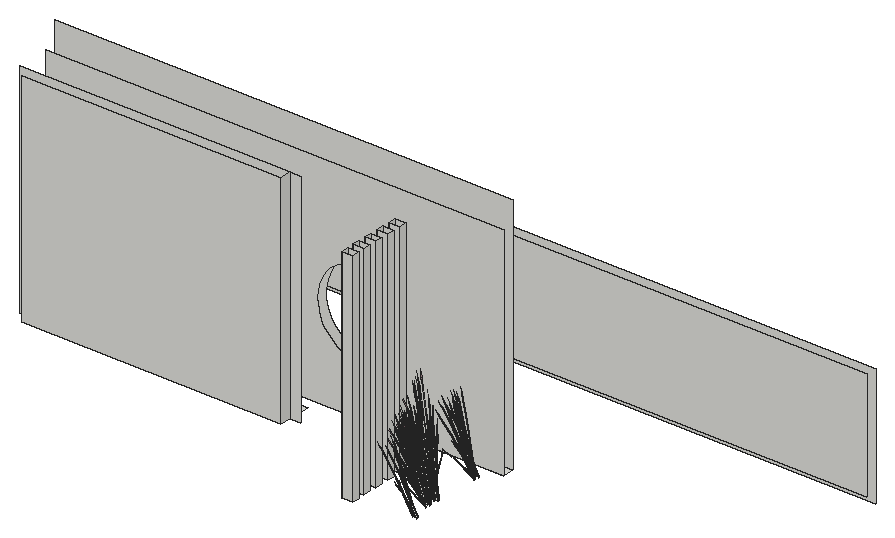
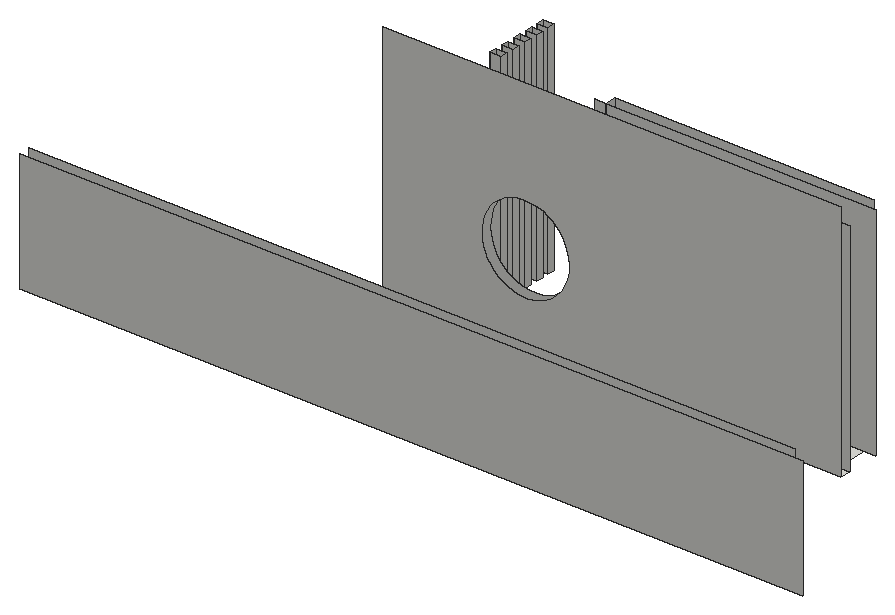
# SketchUp Ruby script. Lengths in inches.
U = 1.inch
M = Sketchup.active_model
def pt(a) = Geom::Point3d.new(a.map { |v| v * U })
def face(e, loops, mat)
  f = e.add_face(loops[0].map { |a| pt(a) })
  loops[1..].each { |l| e.add_face(l.map { |a| pt(a) }).erase! }
  f.material = f.back_material = mat if mat
  f
end
# faces: each face lists its corners as indices into pts; further lists are holes
def faces(e, pts, list, mat = nil) = list.each { |f| face(e, (f[0].is_a?(Array) ? f : [f]).map { |l| l.map { |i| pts[i] } }, mat) }
# xy, xz, yz: faces in a plane at the given z, y or x. An outline is a flat list of corners, or four numbers for a rectangle; further outlines are holes
def ring(l) = l.size == 4 ? [[l[0], l[1]], [l[2], l[1]], [l[2], l[3]], [l[0], l[3]]] : l.each_slice(2).to_a
def flat(e, list, mat, &to3) = list.each { |f| face(e, (f[0].is_a?(Array) ? f : [f]).map { |l| ring(l).map { |u, v| to3.(u, v) } }, mat) }
def xy(e, z, list, mat = nil) = flat(e, list, mat) { |x, y| [x, y, z] }
def xz(e, y, list, mat = nil) = flat(e, list, mat) { |x, z| [x, y, z] }
def yz(e, x, list, mat = nil) = flat(e, list, mat) { |y, z| [x, y, z] }
def lines(e, pts, list) = list.each { |a, b| e.add_line(pt(pts[a]), pt(pts[b])) }
# prism: a flat outline (further loops are holes) pulled along v
def prism(e, loops, v, mat = nil)
  f = face(e, loops, mat); d = Geom::Vector3d.new(v.map { |x| x * U })
  f.pushpull(f.normal.samedirection?(d) ? d.length : -d.length)
end
def box(e, o, s, mat = nil) = prism(e, [[o, [o[0] + s[0], o[1], o[2]], [o[0] + s[0], o[1] + s[1], o[2]], [o[0], o[1] + s[1], o[2]]]], [0, 0, s[2]], mat)
def at(x, y, z, deg = 0) = Geom::Transformation.translation(pt([x, y, z])) * Geom::Transformation.rotation(ORIGIN, Z_AXIS, deg.degrees)
def axes(o, x, y, z) = Geom::Transformation.new([*x, 0, *y, 0, *z, 0, *pt(o).to_a, 1])
def part(name) = M.definitions.add(name)
# library, detail: a bought-in or finely detailed component or shape, given as its bounding box
def library(name, o, s) = part(name).tap { |d| box(d.entities, o, s) }
def detail(e, o, s) = box(e.add_group.entities, o, s)
def put(e, d, t, mat = nil) = e.add_instance(d, t).tap { |i| i.material = mat if mat }
def group(e, t, mat = nil) = e.add_group.tap { |g| g.transformation = t; g.material = mat if mat }.entities
root = M.entities
M.materials.add("LightPink_Translucent").color = [144, 107, 117]
M.materials["LightPink_Translucent"].alpha = 0.75
c1 = part("blade")
p = [[2.15,0.21,22],[0,0.17,0],[0.09,0.45,0],[2.18,0.31,22],[2.29,0.31,22],[0.38,0.45,0],
  [2.48,0.24,33],[2.49,0.24,33],[2.48,0.22,33]]
faces(c1.entities,p,[[0,1,2,3],[4,5,2,3],[6,3,4,7],[8,0,3,6]])
c2 = part("seeds")
p = [[0.3,-0.1,1.38],[-0.01,-0.03,1.59],[-0.01,-0.03,0.03],[0.14,-0.07,-0.07],[0.29,-0.03,3],[0.15,0.01,3.11]]
faces(c2.entities,p,[[0,1,2,3],[1,0,4,5]],"LightPink_Translucent")
c3 = part("blade with seeds")
put(c3.entities,c1,at(0,0,0))
put(c3.entities,c2,axes([2.4,0.25,30.99],[1.5799,-0.05474,1.17369],[-0.12525,1.92788,0.29478],[-0.07173,-0.02425,1.56792]))
xy(root,0,[[51,507,192,519],[45,525,294,531]])
xz(root,467,[[252,0,258,120]])
xz(root,471,[[252,0,258,120]])
xz(root,475,[[252,0,258,120]])
xz(root,479,[[252,0,258,120]])
xz(root,483,[[252,0,258,120]])
xz(root,487,[[252,0,258,120]])
xz(root,491,[[252,0,258,120]])
xz(root,495,[[252,0,258,120]])
xz(root,499,[[252,0,258,120]])
xz(root,501,[[51,0,192,120]])
xz(root,503,[[252,0,258,120]])
xz(root,507,[[45,0,192,120],[192,0,198,120]])
xz(root,525,[[[45,0,294,120],[217.42,27.05,214.41,27.11,211.43,27.55,208.52,28.36,205.74,29.53,203.13,31.04,200.73,32.86,198.58,34.97,196.71,37.33,195.15,39.91,193.92,42.66,193.05,45.54,192.55,48.52,192.42,51.53,192.67,54.53,193.3,57.48,194.29,60.33,195.63,63.03,197.3,65.54,199.27,67.82,201.5,69.83,203.98,71.55,206.65,72.95,209.48,74,212.41,74.69,215.41,75.01,218.42,74.94,221.4,74.5,224.3,73.69,227.08,72.53,229.69,71.02,232.09,69.2,234.25,67.09,236.12,64.73,237.68,62.15,238.91,59.4,239.78,56.51,240.28,53.54,240.41,50.53,240.16,47.52,239.53,44.58,238.54,41.73,237.2,39.03,235.53,36.52,233.5625,34.24,231.32,32.22,228.85,30.5,226.18,29.1,223.35,28.05,220.42,27.36]]])
xz(root,531,[[[45,0,294,132],[217.42,27.05,220.42,27.36,223.35,28.05,226.18,29.1,228.85,30.5,231.32,32.22,233.5625,34.24,235.53,36.52,237.2,39.03,238.54,41.73,239.53,44.58,240.16,47.52,240.41,50.53,240.28,53.54,239.78,56.51,238.91,59.4,237.68,62.15,236.12,64.73,234.25,67.09,232.09,69.2,229.69,71.02,227.08,72.53,224.3,73.69,221.4,74.5,218.42,74.94,215.41,75.01,212.41,74.69,209.48,74,206.65,72.95,203.98,71.55,201.5,69.83,199.27,67.82,197.3,65.54,195.63,63.03,194.29,60.33,193.3,57.48,192.67,54.53,192.42,51.53,192.55,48.52,193.05,45.54,193.92,42.66,195.15,39.91,196.71,37.33,198.58,34.97,200.73,32.86,203.13,31.04,205.74,29.53,208.52,28.36,211.43,27.55,214.41,27.11]]])
xz(root,606.89,[[9,0,426,60]])
xz(root,612.89,[[0,-6,426,60]])
yz(root,192,[[501,0,507,120]])
yz(root,252,[[467,0,471,120],[475,0,479,120],[483,0,487,120],[491,0,495,120],[499,0,503,120]])
yz(root,258,[[467,0,471,120],[475,0,479,120],[483,0,487,120],[491,0,495,120],[499,0,503,120]])
put(root,c3,axes([283.82,485.65,3.875],[0.37107,-0.01478,1.71376],[-0.24616,0.64047,0.13857],[-0.5288,-0.03961,0.73262]))
put(root,c3,axes([283.98,486.78,3.875],[0.31041,-0.13801,1.71376],[0.26133,0.63772,0.13857],[-0.48731,0.14413,0.73262]))
put(root,c3,axes([283.01,487.86,2.59],[0.3109,0.05356,1.43002],[0.20038,0.54709,-0.30754],[-0.42231,0.10241,0.61141]))
put(root,c3,axes([285.76,486.11,3.34],[0.25429,-0.09438,1.77064],[0.08769,0.65901,0.13857],[-0.5508,0.08745,0.63284]))
put(root,c3,axes([283.03,486.55,4.72],[-0.14609,0.08471,1.74944],[0.01243,0.61893,-0.27667],[-0.33486,0.08049,0.14031]))
put(root,c3,axes([284.93,485.05,4.98],[-0.89428,-0.01571,-0.71045],[0.06006,-0.66153,0.08574],[-0.37886,-0.06981,1.00501]))
put(root,c3,axes([284.21,485.22,2.59],[0.17466,0.18165,1.43002],[-0.40248,0.49377,-0.30754],[-0.41327,-0.11802,0.61141]))
put(root,c3,axes([283.49,486.2,4.53],[-0.74348,-0.18202,-0.35414],[0.21685,-0.53102,0.4572],[-0.29933,0.04869,0.87481]))
put(root,c3,axes([284.52,484.62,3.875],[0.3323,0.11241,1.71376],[-0.68769,0.4716,0.13857],[-0.42861,-0.21275,0.73262]))
put(root,c3,axes([281.4,487.18,4.71],[0.11417,0.0175,1.77383],[0.35319,0.57649,-0.16761],[-0.23371,0.15131,0.31391]))
put(root,c3,axes([284,486.47,4.68],[-0.24236,0.59349,-0.51099],[-0.83094,-0.20343,-0.3958],[-0.33455,0.05442,0.97773]))
put(root,c3,axes([284.63,485.1875,4.68],[-0.6496,0.4322,-0.51099],[-0.5689,-0.45657,-0.3958],[-0.33005,-0.06576,0.97773]))
put(root,c3,axes([283.59,486.43,1.49],[0.02269,0.10283,1.76342],[-0.45738,0.53699,-0.26939],[-0.32488,-0.02707,0.30037]))
put(root,c3,axes([283.72,483.98,4.71],[0.06632,0.06511,1.77383],[-0.31973,0.58531,-0.16761],[-0.32381,0.00424,0.31391]))
put(root,c3,axes([282.36,489.01,2.77],[0.37283,-0.29571,1.1486],[0.14711,0.46813,0.84392],[-0.26943,0.08382,0.25299]))
put(root,c3,axes([284.46,483.59,4.72],[-0.19249,-0.00461,1.74944],[-0.61281,0.46055,-0.27667],[-0.32697,-0.0941,0.14031]))
put(root,c3,axes([283.67,486.13,4.73],[0.25275,-0.59491,0.48003],[0.83094,0.20343,0.3958],[-0.32677,0.03575,0.9933]))
put(root,c3,axes([283.96,485.96,5.03],[0.45012,0.59081,-0.1216],[-0.79888,0.29033,-0.67495],[-0.33665,0.07795,1.02557]))
put(root,c3,axes([284.98,484.74,5.03],[-0.0479,0.66354,-0.1216],[-0.90696,-0.01814,-0.67495],[-0.3493,-0.04609,1.02557]))
put(root,c3,axes([284.39,484.78,4.53],[-0.50902,-0.40851,-0.35414],[0.58122,-0.38671,0.4572],[-0.29531,-0.05884,0.87481]))
put(root,c3,axes([283.6,485.98,4.73],[-0.32857,-0.44488,0.0643],[0.59916,-0.21775,0.50621],[-0.26412,0.04296,0.77189]))
put(root,c3,axes([285.11,487.21,3.875],[0.22344,-0.20048,1.71376],[0.56419,0.54113,0.13857],[-0.38697,0.24643,0.73262]))
put(root,c3,axes([283.77,487.73,4.53],[-0.77872,0.09325,-0.35414],[-0.20563,-0.53305,0.4572],[-0.22316,0.14318,0.87481]))
put(root,c3,axes([287.81,479.39,3.875],[0.37107,-0.01478,1.71376],[-0.24616,0.64047,0.13857],[-0.5288,-0.03961,0.73262]))
put(root,c3,axes([283.34,489.3125,1.49],[0.12,0.06519,1.76342],[0.20347,0.60397,-0.26939],[-0.26596,0.12879,0.30037]))
put(root,c3,axes([283.17,485.76,2.77],[0.57115,-0.04669,1.1486],[-0.36229,0.41137,0.84392],[-0.28224,-0.06171,0.25299]))
put(root,c3,axes([283.87,487.62,4.73],[-0.22187,-0.60049,0.48003],[0.87033,-0.10422,0.3958],[-0.25651,0.14123,0.9933]))
put(root,c3,axes([284.32,484.63,5.09],[0.7388,-0.48151,0.53763],[0.63717,0.51135,0.4433],[-0.34662,-0.08882,1.11249]))
put(root,c3,axes([283.7,487.5,4.73],[-0.61415,-0.2744,0.0643],[0.35756,-0.39076,0.50621],[-0.1969,0.12633,0.77189]))
put(root,c3,axes([288.67,511.25,3.875],[0.37107,-0.01478,1.71376],[-0.24616,0.64047,0.13857],[-0.5288,-0.03961,0.73262]))
put(root,c3,axes([284.94,487.7,3.875],[0.16657,-0.22426,1.71376],[0.69879,0.4641,0.13857],[-0.31524,0.28926,0.73262]))
put(root,c3,axes([287.96,480.52,3.875],[0.31041,-0.13801,1.71376],[0.26133,0.63772,0.13857],[-0.48731,0.14413,0.73262]))
put(root,c3,axes([286.99,481.6,2.59],[0.3109,0.05356,1.43002],[0.20038,0.54709,-0.30754],[-0.42231,0.10241,0.61141]))
put(root,c3,axes([284.28,486.14,5.05],[0.74348,0.18202,0.35414],[-0.21685,0.53102,-0.4572],[-0.29933,0.04869,0.87481]))
put(root,c3,axes([284.41,487.79,4.68],[0.22982,0.59576,-0.51099],[-0.87033,0.10422,-0.3958],[-0.24941,0.16002,0.97773]))
put(root,c3,axes([284.65,484.625,4.73],[0.04505,-0.49615,0.0643],[0.68022,0.0136,0.50621],[-0.26056,-0.05192,0.77189]))
put(root,c3,axes([289.74,479.85,3.34],[0.25429,-0.09438,1.77064],[0.08769,0.65901,0.13857],[-0.5508,0.08745,0.63284]))
put(root,c3,axes([283.05,488.86,4.72],[-0.02224,0.12912,1.74944],[0.63107,0.44917,-0.27667],[-0.16521,0.21241,0.14031]))
put(root,c3,axes([286.58,487.37,2.06],[-0.9306,-0.10697,-0.62353],[0.19638,-0.65984,-0.16365],[-0.27771,-0.07995,1.37633]))
put(root,c3,axes([286.75,483.77,5.43],[-0.59706,0.6255,-0.13619],[-0.86465,-0.36036,-0.75594],[-0.30056,-0.17672,1.14864]))
put(root,c3,axes([285.12,485,5.05],[0.50902,0.40851,0.35414],[-0.58122,0.38671,-0.4572],[-0.29531,-0.05884,0.87481]))
put(root,c3,axes([286.49,484.28,4.98],[-0.76283,-0.31537,-0.71045],[0.54213,-0.55263,0.08574],[-0.27638,-0.1883,1.00501]))
put(root,c3,axes([288.82,512.37,3.875],[0.31041,-0.13801,1.71376],[0.26133,0.63772,0.13857],[-0.48731,0.14413,0.73262]))
put(root,c3,axes([286.13,484.29,4.68],[-0.88277,0.1551,-0.51099],[-0.15442,-0.58737,-0.3958],[-0.23711,-0.16832,0.97773]))
put(root,c3,axes([287.86,513.46,2.59],[0.3109,0.05356,1.43002],[0.20038,0.54709,-0.30754],[-0.42231,0.10241,0.61141]))
put(root,c3,axes([287.01,480.29,4.72],[-0.14609,0.08471,1.74944],[0.01243,0.61893,-0.27667],[-0.33486,0.08049,0.14031]))
put(root,c3,axes([288.92,478.79,4.98],[-0.89428,-0.01571,-0.71045],[0.06006,-0.66153,0.08574],[-0.37886,-0.06981,1.00501]))
put(root,c3,axes([285.36,488.62,2.02],[-0.83726,-0.32623,-0.49651],[0.50045,-0.58498,0],[-0.19069,-0.0743,1.57504]))
put(root,c3,axes([284.99,483.76,1.49],[-0.08666,0.08595,1.76342],[-0.87574,0.18531,-0.26939],[-0.21156,-0.16858,0.30037]))
put(root,c3,axes([284,487.37,5.03],[0.82753,0.35977,-0.1216],[-0.47675,0.52101,-0.67495],[-0.2338,0.18111,1.02557]))
put(root,c3,axes([288.2,478.96,2.59],[0.17466,0.18165,1.43002],[-0.40248,0.49377,-0.30754],[-0.41327,-0.11802,0.61141]))
put(root,c3,axes([285.87,489.01,2.375],[-0.55932,0.6538,0],[-0.93577,-0.36461,-0.51607],[-0.21313,-0.08304,1.63711]))
put(root,c3,axes([290.61,511.71,3.34],[0.25429,-0.09438,1.77064],[0.08769,0.65901,0.13857],[-0.5508,0.08745,0.63284]))
put(root,c3,axes([287.48,479.9375,4.53],[-0.74348,-0.18202,-0.35414],[0.21685,-0.53102,0.4572],[-0.29933,0.04869,0.87481]))
put(root,c3,axes([288.51,478.36,3.875],[0.3323,0.11241,1.71376],[-0.68769,0.4716,0.13857],[-0.42861,-0.21275,0.73262]))
put(root,c3,axes([290.35,467.61,3.875],[0.37107,-0.01478,1.71376],[-0.24616,0.64047,0.13857],[-0.5288,-0.03961,0.73262]))
put(root,c3,axes([282.63,488.93,5.65],[0.78943,0.17416,-0.06488],[-0.24284,0.53604,-0.29416],[-0.12912,0.08139,0.97024]))
put(root,c3,axes([285.39,480.92,4.71],[0.11417,0.0175,1.77383],[0.35319,0.57649,-0.16761],[-0.23371,0.15131,0.31391]))
put(root,c3,axes([287.99,480.21,4.68],[-0.24236,0.59349,-0.51099],[-0.83094,-0.20343,-0.3958],[-0.33455,0.05442,0.97773]))
put(root,c3,axes([284.4,487.42,5.05],[0.77872,-0.09325,0.35414],[0.20563,0.53305,-0.4572],[-0.22316,0.14318,0.87481]))
put(root,c3,axes([288.62,478.93,4.68],[-0.6496,0.4322,-0.51099],[-0.5689,-0.45657,-0.3958],[-0.33005,-0.06576,0.97773]))
put(root,c3,axes([287.875,512.15,4.72],[-0.14609,0.08471,1.74944],[0.01243,0.61893,-0.27667],[-0.33486,0.08049,0.14031]))
put(root,c3,axes([287.57,480.17,1.49],[0.02269,0.10283,1.76342],[-0.45738,0.53699,-0.26939],[-0.32488,-0.02707,0.30037]))
put(root,c3,axes([284.85,489.96,2.59],[0.28231,-0.10293,1.43002],[0.69701,0.31035,-0.30754],[-0.20746,0.26854,0.61141]))
put(root,c3,axes([289.78,510.65,4.98],[-0.89428,-0.01571,-0.71045],[0.06006,-0.66153,0.08574],[-0.37886,-0.06981,1.00501]))
put(root,c3,axes([284.45,484.09,2.13],[-0.25807,0.53277,-0.03893],[-0.79428,-0.16389,-0.17649],[-0.1206,-0.08714,0.58215]))
put(root,c3,axes([289.06,510.8125,2.59],[0.17466,0.18165,1.43002],[-0.40248,0.49377,-0.30754],[-0.41327,-0.11802,0.61141]))
put(root,c3,axes([287.7,477.72,4.71],[0.06632,0.06511,1.77383],[-0.31973,0.58531,-0.16761],[-0.32381,0.00424,0.31391]))
put(root,c3,axes([288.34,511.8,4.53],[-0.74348,-0.18202,-0.35414],[0.21685,-0.53102,0.4572],[-0.29933,0.04869,0.87481]))
put(root,c3,axes([286.52,482.28,4.71],[-0.01669,0.07821,1.77383],[-0.82314,0.28383,-0.16761],[-0.24223,-0.14508,0.31391]))
put(root,c3,axes([289.37,510.22,3.875],[0.3323,0.11241,1.71376],[-0.68769,0.4716,0.13857],[-0.42861,-0.21275,0.73262]))
put(root,c3,axes([286.35,482.75,2.77],[0.37283,-0.29571,1.1486],[0.14711,0.46813,0.84392],[-0.26943,0.08382,0.25299]))
put(root,c3,axes([285.63,483.42,2.59],[-0.05417,0.21344,1.43002],[-0.79196,0.17867,-0.30754],[-0.18512,-0.27588,0.61141]))
put(root,c3,axes([288.44,477.33,4.72],[-0.19249,-0.00461,1.74944],[-0.61281,0.46055,-0.27667],[-0.32697,-0.0941,0.14031]))
put(root,c3,axes([285.89,483.97,3.875],[0.2045,0.20949,1.71376],[-0.94495,0.17636,0.13857],[-0.21357,-0.32887,0.73262]))
put(root,c3,axes([287.63,487.46,2.67],[-0.90324,0.43318,-0.29095],[-0.60064,-0.61207,-0.50002],[-0.22285,-0.06216,1.59708]))
put(root,c3,axes([290.51,468.74,3.875],[0.31041,-0.13801,1.71376],[0.26133,0.63772,0.13857],[-0.48731,0.14413,0.73262]))
put(root,c3,axes([285.14,488.83,4.73],[-0.63704,-0.44518,0.48003],[0.67652,-0.38394,0.3958],[-0.11751,0.20886,0.9933]))
put(root,c3,axes([286.25,512.77,4.71],[0.11417,0.0175,1.77383],[0.35319,0.57649,-0.16761],[-0.23371,0.15131,0.31391]))
put(root,c3,axes([287.65,479.875,4.73],[0.25275,-0.59491,0.48003],[0.83094,0.20343,0.3958],[-0.32677,0.03575,0.9933]))
put(root,c3,axes([288.85,512.07,4.68],[-0.24236,0.59349,-0.51099],[-0.83094,-0.20343,-0.3958],[-0.33455,0.05442,0.97773]))
put(root,c3,axes([287.95,479.7,5.03],[0.45012,0.59081,-0.1216],[-0.79888,0.29033,-0.67495],[-0.33665,0.07795,1.02557]))
put(root,c3,axes([286.22,483.86,4.53],[-0.13817,-0.52554,-0.35414],[0.78985,-0.13877,0.4572],[-0.21215,-0.1506,0.87481]))
put(root,c3,axes([288.96,478.47,5.03],[-0.0479,0.66354,-0.1216],[-0.90696,-0.01814,-0.67495],[-0.3493,-0.04609,1.02557]))
put(root,c3,axes([289.54,469.82,2.59],[0.3109,0.05356,1.43002],[0.20038,0.54709,-0.30754],[-0.42231,0.10241,0.61141]))
put(root,c3,axes([284.02,486.52,2.375],[-1.11865,0,0],[0,-0.72922,-0.51607],[0,-0.16609,1.63711]))
put(root,c3,axes([285.59,488.37,2.03],[-0.21015,-0.56852,-0.30978],[0.83462,-0.16144,0.30978],[-0.16826,-0.06556,1.38974]))
put(root,c3,axes([288.38,478.52,4.53],[-0.50902,-0.40851,-0.35414],[0.58122,-0.38671,0.4572],[-0.29531,-0.05884,0.87481]))
put(root,c3,axes([289.48,510.78,4.68],[-0.6496,0.4322,-0.51099],[-0.5689,-0.45657,-0.3958],[-0.33005,-0.06576,0.97773]))
put(root,c3,axes([284.9,488.79,4.73],[-0.73517,-0.0304,0.0643],[0.02016,-0.45906,0.50621],[-0.07693,0.17585,0.77189]))
put(root,c3,axes([287.59,479.72,4.73],[-0.32857,-0.44488,0.0643],[0.59916,-0.21775,0.50621],[-0.26412,0.04296,0.77189]))
put(root,c3,axes([288.4375,512.03,1.49],[0.02269,0.10283,1.76342],[-0.45738,0.53699,-0.26939],[-0.32488,-0.02707,0.30037]))
put(root,c3,axes([289.1,480.95,3.875],[0.22344,-0.20048,1.71376],[0.56419,0.54113,0.13857],[-0.38697,0.24643,0.73262]))
put(root,c3,axes([287.75,481.47,4.53],[-0.77872,0.09325,-0.35414],[-0.20563,-0.53305,0.4572],[-0.22316,0.14318,0.87481]))
put(root,c3,axes([285.14,488.97,4.53],[-0.60531,0.34352,-0.35414],[-0.573,-0.39225,0.4572],[-0.08718,0.19929,0.87481]))
put(root,c3,axes([292.29,468.07,3.34],[0.25429,-0.09438,1.77064],[0.08769,0.65901,0.13857],[-0.5508,0.08745,0.63284]))
put(root,c3,axes([287.33,483.05,1.49],[0.12,0.06519,1.76342],[0.20347,0.60397,-0.26939],[-0.26596,0.12879,0.30037]))
put(root,c3,axes([288.57,509.57,4.71],[0.06632,0.06511,1.77383],[-0.31973,0.58531,-0.16761],[-0.32381,0.00424,0.31391]))
put(root,c3,axes([287.16,479.5,2.77],[0.57115,-0.04669,1.1486],[-0.36229,0.41137,0.84392],[-0.28224,-0.06171,0.25299]))
put(root,c3,axes([288.23,487.9375,2.06],[-0.60257,0.49041,-0.62353],[-0.74854,-0.44469,-0.16365],[-0.24146,0.12234,1.37633]))
put(root,c3,axes([286.6875,484.29,5.05],[0.13817,0.52554,0.35414],[-0.78985,0.13877,-0.4572],[-0.21215,-0.1506,0.87481]))
put(root,c3,axes([287.21,514.61,2.77],[0.37283,-0.29571,1.1486],[0.14711,0.46813,0.84392],[-0.26943,0.08382,0.25299]))
put(root,c3,axes([282.98,490.1875,4.71],[0.10149,-0.03939,1.77383],[0.83886,0.26202,-0.16761],[-0.01971,0.21816,0.31391]))
put(root,c3,axes([289.31,509.18,4.72],[-0.19249,-0.00461,1.74944],[-0.61281,0.46055,-0.27667],[-0.32697,-0.0941,0.14031]))
put(root,c3,axes([284.89,486.33,2.33],[-0.83213,0.54855,0.30756],[-0.83263,-0.54278,-0.36492],[-0.02906,-0.15578,1.64885]))
put(root,c3,axes([287.85,481.36,4.73],[-0.22187,-0.60049,0.48003],[0.87033,-0.10422,0.3958],[-0.25651,0.14123,0.9933]))
put(root,c3,axes([288.3125,487.84,3.33],[0.77308,0.2631,1.51261],[-0.75736,0.56681,0.59816],[-0.33924,-0.33594,1.26806]))
put(root,c3,axes([288.52,511.73,4.73],[0.25275,-0.59491,0.48003],[0.83094,0.20343,0.3958],[-0.32677,0.03575,0.9933]))
put(root,c3,axes([288.8125,511.56,5.03],[0.45012,0.59081,-0.1216],[-0.79888,0.29033,-0.67495],[-0.33665,0.07795,1.02557]))
put(root,c3,axes([288.3,478.37,5.09],[0.7388,-0.48151,0.53763],[0.63717,0.51135,0.4433],[-0.34662,-0.08882,1.11249]))
put(root,c3,axes([289.82,510.33,5.03],[-0.0479,0.66354,-0.1216],[-0.90696,-0.01814,-0.67495],[-0.3493,-0.04609,1.02557]))
put(root,c3,axes([285.36,483.07,2.77],[0.46666,0.22709,1.1486],[-0.67962,0.13651,0.84392],[-0.14541,-0.17452,0.25299]))
put(root,c3,axes([288.65,487.66,2.46],[-0.87356,-0.52515,-0.25192],[0.73507,-0.5897,0.5513],[-0.23523,0.06143,1.68216]))
put(root,c3,axes([289.24,510.38,4.53],[-0.50902,-0.40851,-0.35414],[0.58122,-0.38671,0.4572],[-0.29531,-0.05884,0.87481]))
put(root,c3,axes([289.56,468.51,4.72],[-0.14609,0.08471,1.74944],[0.01243,0.61893,-0.27667],[-0.33486,0.08049,0.14031]))
